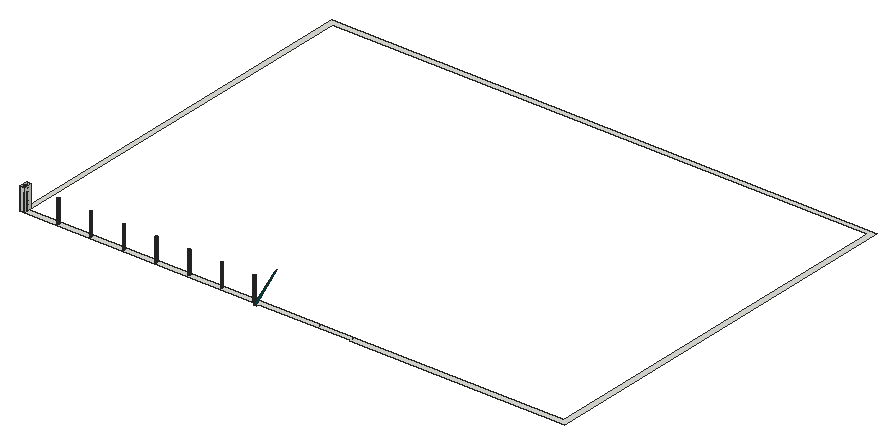
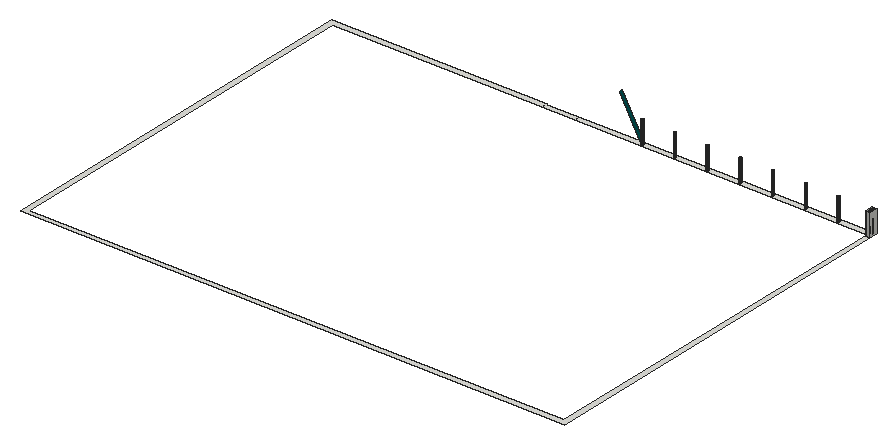
# SketchUp Ruby script. Lengths in inches.
U = 1.inch
M = Sketchup.active_model
def pt(a) = Geom::Point3d.new(a.map { |v| v * U })
def face(e, loops, mat)
  f = e.add_face(loops[0].map { |a| pt(a) })
  loops[1..].each { |l| e.add_face(l.map { |a| pt(a) }).erase! }
  f.material = f.back_material = mat if mat
  f
end
# faces: each face lists its corners as indices into pts; further lists are holes
def faces(e, pts, list, mat = nil) = list.each { |f| face(e, (f[0].is_a?(Array) ? f : [f]).map { |l| l.map { |i| pts[i] } }, mat) }
# xy, xz, yz: faces in a plane at the given z, y or x. An outline is a flat list of corners, or four numbers for a rectangle; further outlines are holes
def ring(l) = l.size == 4 ? [[l[0], l[1]], [l[2], l[1]], [l[2], l[3]], [l[0], l[3]]] : l.each_slice(2).to_a
def flat(e, list, mat, &to3) = list.each { |f| face(e, (f[0].is_a?(Array) ? f : [f]).map { |l| ring(l).map { |u, v| to3.(u, v) } }, mat) }
def xy(e, z, list, mat = nil) = flat(e, list, mat) { |x, y| [x, y, z] }
def xz(e, y, list, mat = nil) = flat(e, list, mat) { |x, z| [x, y, z] }
def yz(e, x, list, mat = nil) = flat(e, list, mat) { |y, z| [x, y, z] }
def lines(e, pts, list) = list.each { |a, b| e.add_line(pt(pts[a]), pt(pts[b])) }
# prism: a flat outline (further loops are holes) pulled along v
def prism(e, loops, v, mat = nil)
  f = face(e, loops, mat); d = Geom::Vector3d.new(v.map { |x| x * U })
  f.pushpull(f.normal.samedirection?(d) ? d.length : -d.length)
end
def box(e, o, s, mat = nil) = prism(e, [[o, [o[0] + s[0], o[1], o[2]], [o[0] + s[0], o[1] + s[1], o[2]], [o[0], o[1] + s[1], o[2]]]], [0, 0, s[2]], mat)
def at(x, y, z, deg = 0) = Geom::Transformation.translation(pt([x, y, z])) * Geom::Transformation.rotation(ORIGIN, Z_AXIS, deg.degrees)
def axes(o, x, y, z) = Geom::Transformation.new([*x, 0, *y, 0, *z, 0, *pt(o).to_a, 1])
def part(name) = M.definitions.add(name)
# library, detail: a bought-in or finely detailed component or shape, given as its bounding box
def library(name, o, s) = part(name).tap { |d| box(d.entities, o, s) }
def detail(e, o, s) = box(e.add_group.entities, o, s)
def put(e, d, t, mat = nil) = e.add_instance(d, t).tap { |i| i.material = mat if mat }
def group(e, t, mat = nil) = e.add_group.tap { |g| g.transformation = t; g.material = mat if mat }.entities
root = M.entities
M.materials.add("[0136_Charcoal]").color = [35, 35, 35]
M.materials.add("[Color H08]").color = [0, 102, 102]
xy(root,420,[[[426.66,30,430.89,30,430.89,36,595.0625,36,595.0625,35.0625,982.625,35.0625,982.625,738,0,738,0,49.95,8.62,49.95,8.62,36,426.66,36],[604.0625,44.0625,604.0625,45,9,45,9,729,973.625,729,973.625,44.0625],[973.58,39.3,973.09,39.36,972.64,39.55,972.25,39.85,971.96,40.24,971.77,40.6875,971.7,41.17,971.77,41.66,971.96,42.11,972.25,42.5,972.64,42.8,973.09,42.98,973.58,43.05,974.06,42.98,974.52,42.8,974.91,42.5,975.2,42.11,975.39,41.66,975.45,41.17,975.39,40.6875,975.2,40.24,974.91,39.85,974.52,39.55,974.06,39.36],[890.27,39.3,889.78,39.36,889.33,39.55,888.94,39.85,888.64,40.24,888.46,40.6875,888.39,41.17,888.46,41.66,888.64,42.11,888.94,42.5,889.33,42.8,889.78,42.98,890.27,43.05,890.75,42.98,891.2,42.8,891.59,42.5,891.89,42.11,892.08,41.66,892.14,41.17,892.08,40.6875,891.89,40.24,891.59,39.85,891.2,39.55,890.75,39.36],[831.27,39.3,830.78,39.36,830.33,39.55,829.94,39.85,829.64,40.24,829.46,40.6875,829.39,41.17,829.46,41.66,829.64,42.11,829.94,42.5,830.33,42.8,830.78,42.98,831.27,43.05,831.75,42.98,832.2,42.8,832.59,42.5,832.89,42.11,833.08,41.66,833.14,41.17,833.08,40.6875,832.89,40.24,832.59,39.85,832.2,39.55,831.75,39.36],[772.27,39.3,771.78,39.36,771.33,39.55,770.94,39.85,770.64,40.24,770.46,40.6875,770.39,41.17,770.46,41.66,770.64,42.11,770.94,42.5,771.33,42.8,771.78,42.98,772.27,43.05,772.75,42.98,773.2,42.8,773.59,42.5,773.89,42.11,774.08,41.66,774.14,41.17,774.08,40.6875,773.89,40.24,773.59,39.85,773.2,39.55,772.75,39.36],[713.27,39.3,712.78,39.36,712.33,39.55,711.94,39.85,711.64,40.24,711.46,40.6875,711.39,41.17,711.46,41.66,711.64,42.11,711.94,42.5,712.33,42.8,712.78,42.98,713.27,43.05,713.75,42.98,714.2,42.8,714.59,42.5,714.89,42.11,715.08,41.66,715.14,41.17,715.08,40.6875,714.89,40.24,714.59,39.85,714.2,39.55,713.75,39.36],[654.27,39.3,653.78,39.36,653.33,39.55,652.94,39.85,652.64,40.24,652.46,40.6875,652.39,41.17,652.46,41.66,652.64,42.11,652.94,42.5,653.33,42.8,653.78,42.98,654.27,43.05,654.75,42.98,655.2,42.8,655.59,42.5,655.89,42.11,656.08,41.66,656.14,41.17,656.08,40.6875,655.89,40.24,655.59,39.85,655.2,39.55,654.75,39.36],[595.27,39.3,594.78,39.36,594.33,39.55,593.94,39.85,593.64,40.24,593.46,40.6875,593.39,41.17,593.46,41.66,593.64,42.11,593.94,42.5,594.33,42.8,594.78,42.98,595.27,43.05,595.75,42.98,596.2,42.8,596.59,42.5,596.89,42.11,597.08,41.66,597.14,41.17,597.08,40.6875,596.89,40.24,596.59,39.85,596.2,39.55,595.75,39.36],[536.27,39.3,535.78,39.36,535.33,39.55,534.94,39.85,534.64,40.24,534.46,40.6875,534.39,41.17,534.46,41.66,534.64,42.11,534.94,42.5,535.33,42.8,535.78,42.98,536.27,43.05,536.75,42.98,537.2,42.8,537.59,42.5,537.89,42.11,538.08,41.66,538.14,41.17,538.08,40.6875,537.89,40.24,537.59,39.85,537.2,39.55,536.75,39.36],[477.27,39.3,476.78,39.36,476.33,39.55,475.94,39.85,475.64,40.24,475.46,40.6875,475.39,41.17,475.46,41.66,475.64,42.11,475.94,42.5,476.33,42.8,476.78,42.98,477.27,43.05,477.75,42.98,478.2,42.8,478.59,42.5,478.89,42.11,479.08,41.66,479.14,41.17,479.08,40.6875,478.89,40.24,478.59,39.85,478.2,39.55,477.75,39.36],[418.27,39.3,417.78,39.36,417.33,39.55,416.94,39.85,416.64,40.24,416.46,40.6875,416.39,41.17,416.46,41.66,416.64,42.11,416.94,42.5,417.33,42.8,417.78,42.98,418.27,43.05,418.75,42.98,419.2,42.8,419.59,42.5,419.89,42.11,420.08,41.66,420.14,41.17,420.08,40.6875,419.89,40.24,419.59,39.85,419.2,39.55,418.75,39.36],[359.27,39.3,358.78,39.36,358.33,39.55,357.94,39.85,357.64,40.24,357.46,40.6875,357.39,41.17,357.46,41.66,357.64,42.11,357.94,42.5,358.33,42.8,358.78,42.98,359.27,43.05,359.75,42.98,360.2,42.8,360.59,42.5,360.89,42.11,361.08,41.66,361.14,41.17,361.08,40.6875,360.89,40.24,360.59,39.85,360.2,39.55,359.75,39.36],[300.27,39.3,299.78,39.36,299.33,39.55,298.94,39.85,298.64,40.24,298.46,40.6875,298.39,41.17,298.46,41.66,298.64,42.11,298.94,42.5,299.33,42.8,299.78,42.98,300.27,43.05,300.75,42.98,301.2,42.8,301.59,42.5,301.89,42.11,302.08,41.66,302.14,41.17,302.08,40.6875,301.89,40.24,301.59,39.85,301.2,39.55,300.75,39.36],[241.27,39.3,240.78,39.36,240.33,39.55,239.94,39.85,239.64,40.24,239.46,40.6875,239.39,41.17,239.46,41.66,239.64,42.11,239.94,42.5,240.33,42.8,240.78,42.98,241.27,43.05,241.75,42.98,242.2,42.8,242.59,42.5,242.89,42.11,243.08,41.66,243.14,41.17,243.08,40.6875,242.89,40.24,242.59,39.85,242.2,39.55,241.75,39.36],[182.27,39.3,181.78,39.36,181.33,39.55,180.94,39.85,180.64,40.24,180.46,40.6875,180.39,41.17,180.46,41.66,180.64,42.11,180.94,42.5,181.33,42.8,181.78,42.98,182.27,43.05,182.75,42.98,183.2,42.8,183.59,42.5,183.89,42.11,184.08,41.66,184.14,41.17,184.08,40.6875,183.89,40.24,183.59,39.85,183.2,39.55,182.75,39.36],[123.27,39.3,122.78,39.36,122.33,39.55,121.94,39.85,121.64,40.24,121.46,40.6875,121.39,41.17,121.46,41.66,121.64,42.11,121.94,42.5,122.33,42.8,122.78,42.98,123.27,43.05,123.75,42.98,124.2,42.8,124.59,42.5,124.89,42.11,125.08,41.66,125.14,41.17,125.08,40.6875,124.89,40.24,124.59,39.85,124.2,39.55,123.75,39.36],[64.27,39.3,63.78,39.36,63.33,39.55,62.94,39.85,62.64,40.24,62.46,40.6875,62.39,41.17,62.46,41.66,62.64,42.11,62.94,42.5,63.33,42.8,63.78,42.98,64.27,43.05,64.75,42.98,65.2,42.8,65.59,42.5,65.89,42.11,66.08,41.66,66.14,41.17,66.08,40.6875,65.89,40.24,65.59,39.85,65.2,39.55,64.75,39.36]],[[0,36,8.62,49.95],[5.27,39.3,5.75,39.36,6.2,39.55,6.59,39.85,6.89,40.24,7.08,40.6875,7.14,41.17,7.08,41.66,6.89,42.11,6.59,42.5,6.2,42.8,5.75,42.98,5.27,43.05,4.78,42.98,4.33,42.8,3.94,42.5,3.64,42.11,3.46,41.66,3.39,41.17,3.46,40.6875,3.64,40.24,3.94,39.85,4.33,39.55,4.78,39.36]],[64.27,39.3,63.78,39.36,63.33,39.55,62.94,39.85,62.64,40.24,62.46,40.6875,62.39,41.17,62.46,41.66,62.64,42.11,62.94,42.5,63.33,42.8,63.78,42.98,64.27,43.05,64.75,42.98,65.2,42.8,65.59,42.5,65.89,42.11,66.08,41.66,66.14,41.17,66.08,40.6875,65.89,40.24,65.59,39.85,65.2,39.55,64.75,39.36],[123.27,39.3,122.78,39.36,122.33,39.55,121.94,39.85,121.64,40.24,121.46,40.6875,121.39,41.17,121.46,41.66,121.64,42.11,121.94,42.5,122.33,42.8,122.78,42.98,123.27,43.05,123.75,42.98,124.2,42.8,124.59,42.5,124.89,42.11,125.08,41.66,125.14,41.17,125.08,40.6875,124.89,40.24,124.59,39.85,124.2,39.55,123.75,39.36],[182.27,39.3,181.78,39.36,181.33,39.55,180.94,39.85,180.64,40.24,180.46,40.6875,180.39,41.17,180.46,41.66,180.64,42.11,180.94,42.5,181.33,42.8,181.78,42.98,182.27,43.05,182.75,42.98,183.2,42.8,183.59,42.5,183.89,42.11,184.08,41.66,184.14,41.17,184.08,40.6875,183.89,40.24,183.59,39.85,183.2,39.55,182.75,39.36],
  [241.27,39.3,240.78,39.36,240.33,39.55,239.94,39.85,239.64,40.24,239.46,40.6875,239.39,41.17,239.46,41.66,239.64,42.11,239.94,42.5,240.33,42.8,240.78,42.98,241.27,43.05,241.75,42.98,242.2,42.8,242.59,42.5,242.89,42.11,243.08,41.66,243.14,41.17,243.08,40.6875,242.89,40.24,242.59,39.85,242.2,39.55,241.75,39.36],[300.27,39.3,299.78,39.36,299.33,39.55,298.94,39.85,298.64,40.24,298.46,40.6875,298.39,41.17,298.46,41.66,298.64,42.11,298.94,42.5,299.33,42.8,299.78,42.98,300.27,43.05,300.75,42.98,301.2,42.8,301.59,42.5,301.89,42.11,302.08,41.66,302.14,41.17,302.08,40.6875,301.89,40.24,301.59,39.85,301.2,39.55,300.75,39.36],[359.27,39.3,358.78,39.36,358.33,39.55,357.94,39.85,357.64,40.24,357.46,40.6875,357.39,41.17,357.46,41.66,357.64,42.11,357.94,42.5,358.33,42.8,358.78,42.98,359.27,43.05,359.75,42.98,360.2,42.8,360.59,42.5,360.89,42.11,361.08,41.66,361.14,41.17,361.08,40.6875,360.89,40.24,360.59,39.85,360.2,39.55,359.75,39.36],[418.27,39.3,417.78,39.36,417.33,39.55,416.94,39.85,416.64,40.24,416.46,40.6875,416.39,41.17,416.46,41.66,416.64,42.11,416.94,42.5,417.33,42.8,417.78,42.98,418.27,43.05,418.75,42.98,419.2,42.8,419.59,42.5,419.89,42.11,420.08,41.66,420.14,41.17,420.08,40.6875,419.89,40.24,419.59,39.85,419.2,39.55,418.75,39.36]])
xz(root,36,[[0,420,8.62,460.3125]])
xz(root,49.95,[[0,420,8.62,460.3125]])
yz(root,0,[[36,420,49.95,460.3125]])
yz(root,8.62,[[[36,420,49.95,460.3125],[41.84,455.4,41.36,455.46,40.91,455.65,40.52,455.95,40.22,456.34,40.03,456.79,39.97,457.28,40.03,457.76,40.22,458.21,40.52,458.6,40.91,458.9,41.36,459.09,41.84,459.15,42.33,459.09,42.78,458.9,43.17,458.6,43.47,458.21,43.66,457.76,43.72,457.28,43.66,456.79,43.47,456.34,43.17,455.95,42.78,455.65,42.33,455.46],[41.84,448.46,41.36,448.53,40.91,448.71,40.52,449.01,40.22,449.4,40.03,449.85,39.97,450.34,40.03,450.82,40.22,451.28,40.52,451.66,40.91,451.96,41.36,452.15,41.84,452.21,42.33,452.15,42.78,451.96,43.17,451.66,43.47,451.28,43.66,450.82,43.72,450.34,43.66,449.85,43.47,449.4,43.17,449.01,42.78,448.71,42.33,448.53],[41.84,441.53,41.36,441.59,40.91,441.78,40.52,442.07,40.22,442.46,40.03,442.92,39.97,443.4,40.03,443.89,40.22,444.34,40.52,444.73,40.91,445.02,41.36,445.21,41.84,445.28,42.33,445.21,42.78,445.02,43.17,444.73,43.47,444.34,43.66,443.89,43.72,443.4,43.66,442.92,43.47,442.46,43.17,442.07,42.78,441.78,42.33,441.59],[41.84,434.59,41.36,434.65,40.91,434.84,40.52,435.14,40.22,435.53,40.03,435.98,39.97,436.46,40.03,436.95,40.22,437.4,40.52,437.79,40.91,438.09,41.36,438.27,41.84,438.34,42.33,438.27,42.78,438.09,43.17,437.79,43.47,437.4,43.66,436.95,43.72,436.46,43.66,435.98,43.47,435.53,43.17,435.14,42.78,434.84,42.33,434.65],[41.84,427.65,41.36,427.71,40.91,427.9,40.52,428.2,40.22,428.59,40.03,429.04,39.97,429.53,40.03,430.01,40.22,430.46,40.52,430.85,40.91,431.15,41.36,431.34,41.84,431.4,42.33,431.34,42.78,431.15,43.17,430.85,43.47,430.46,43.66,430.01,43.72,429.53,43.66,429.04,43.47,428.59,43.17,428.2,42.78,427.9,42.33,427.71],[41.84,420.71,41.36,420.78,40.91,420.96,40.52,421.26,40.22,421.65,40.03,422.1,39.97,422.59,40.03,423.07,40.22,423.53,40.52,423.91,40.91,424.21,41.36,424.4,41.84,424.46,42.33,424.4,42.78,424.21,43.17,423.91,43.47,423.53,43.66,423.07,43.72,422.59,43.66,422.1,43.47,421.65,43.17,421.26,42.78,420.96,42.33,420.78]]])
p = [[463.18,36,486.6875],[426.66,36,420],[426.66,30,420],[463.18,30,486.6875],[4.78,39.36,420],[5.27,39.3,420],
  [5.27,39.3,460.3125],[4.78,39.36,460.3125],[5.75,39.36,420],[5.75,39.36,460.3125],[63.78,39.36,420],[64.27,39.3,420],
  [64.27,39.3,460.3125],[63.78,39.36,460.3125],[64.75,39.36,420],[64.75,39.36,460.3125],[122.78,39.36,420],[123.27,39.3,420],
  [123.27,39.3,460.3125],[122.78,39.36,460.3125],[123.75,39.36,420],[123.75,39.36,460.3125],[181.78,39.36,420],[182.27,39.3,420],
  [182.27,39.3,460.3125],[181.78,39.36,460.3125],[182.75,39.36,420],[182.75,39.36,460.3125],[240.78,39.36,420],[241.27,39.3,420],
  [241.27,39.3,460.3125],[240.78,39.36,460.3125],[241.75,39.36,420],[241.75,39.36,460.3125],[299.78,39.36,420],[300.27,39.3,420],
  [300.27,39.3,460.3125],[299.78,39.36,460.3125],[300.75,39.36,420],[300.75,39.36,460.3125],[358.78,39.36,420],[359.27,39.3,420],
  [359.27,39.3,460.3125],[358.78,39.36,460.3125],[359.75,39.36,420],[359.75,39.36,460.3125],[417.78,39.36,420],[418.27,39.3,420],
  [418.27,39.3,460.3125],[417.78,39.36,460.3125],[418.75,39.36,420],[418.75,39.36,460.3125],[4.33,39.55,420],[4.33,39.55,460.3125],
  [6.2,39.55,420],[6.2,39.55,460.3125],[63.33,39.55,420],[63.33,39.55,460.3125],[65.2,39.55,420],[65.2,39.55,460.3125],
  [122.33,39.55,420],[122.33,39.55,460.3125],[124.2,39.55,420],[124.2,39.55,460.3125],[181.33,39.55,420],[181.33,39.55,460.3125],
  [183.2,39.55,420],[183.2,39.55,460.3125],[240.33,39.55,420],[240.33,39.55,460.3125],[242.2,39.55,420],[242.2,39.55,460.3125],
  [299.33,39.55,420],[299.33,39.55,460.3125],[301.2,39.55,420],[301.2,39.55,460.3125],[358.33,39.55,420],[358.33,39.55,460.3125],
  [360.2,39.55,420],[360.2,39.55,460.3125],[417.33,39.55,420],[417.33,39.55,460.3125],[419.2,39.55,420],[419.2,39.55,460.3125],
  [3.94,39.85,420],[3.94,39.85,460.3125],[6.59,39.85,420],[6.59,39.85,460.3125],[62.94,39.85,420],[62.94,39.85,460.3125],
  [65.59,39.85,420],[65.59,39.85,460.3125],[121.94,39.85,420],[121.94,39.85,460.3125],[124.59,39.85,420],[124.59,39.85,460.3125],
  [180.94,39.85,420],[180.94,39.85,460.3125],[183.59,39.85,420],[183.59,39.85,460.3125],[239.94,39.85,420],[239.94,39.85,460.3125],
  [242.59,39.85,420],[242.59,39.85,460.3125],[298.94,39.85,420],[298.94,39.85,460.3125],[301.59,39.85,420],[301.59,39.85,460.3125],
  [357.94,39.85,420],[357.94,39.85,460.3125],[360.59,39.85,420],[360.59,39.85,460.3125],[416.94,39.85,420],[416.94,39.85,460.3125],
  [419.59,39.85,420],[419.59,39.85,460.3125],[3.64,40.24,420],[3.64,40.24,460.3125],[6.89,40.24,420],[6.89,40.24,460.3125],
  [62.64,40.24,420],[62.64,40.24,460.3125],[65.89,40.24,420],[65.89,40.24,460.3125],[121.64,40.24,420],[121.64,40.24,460.3125],
  [124.89,40.24,420],[124.89,40.24,460.3125],[180.64,40.24,420],[180.64,40.24,460.3125],[183.89,40.24,420],[183.89,40.24,460.3125],
  [239.64,40.24,420],[239.64,40.24,460.3125],[242.89,40.24,420],[242.89,40.24,460.3125],[298.64,40.24,420],[298.64,40.24,460.3125],
  [301.89,40.24,420],[301.89,40.24,460.3125],[357.64,40.24,420],[357.64,40.24,460.3125],[360.89,40.24,420],[360.89,40.24,460.3125],
  [416.64,40.24,420],[416.64,40.24,460.3125],[419.89,40.24,420],[419.89,40.24,460.3125],[3.46,40.6875,420],[3.46,40.6875,460.3125],
  [7.08,40.6875,420],[7.08,40.6875,460.3125],[62.46,40.6875,420],[62.46,40.6875,460.3125],[66.08,40.6875,420],[66.08,40.6875,460.3125],
  [121.46,40.6875,420],[121.46,40.6875,460.3125],[125.08,40.6875,420],[125.08,40.6875,460.3125],[180.46,40.6875,420],[180.46,40.6875,460.3125],
  [184.08,40.6875,420],[184.08,40.6875,460.3125],[239.46,40.6875,420],[239.46,40.6875,460.3125],[243.08,40.6875,420],[243.08,40.6875,460.3125],
  [298.46,40.6875,420],[298.46,40.6875,460.3125],[302.08,40.6875,420],[302.08,40.6875,460.3125],[357.46,40.6875,420],[357.46,40.6875,460.3125],
  [361.08,40.6875,420],[361.08,40.6875,460.3125],[416.46,40.6875,420],[416.46,40.6875,460.3125],[420.08,40.6875,420],[420.08,40.6875,460.3125],
  [3.39,41.17,420],[3.39,41.17,460.3125],[7.14,41.17,420],[7.14,41.17,460.3125],[62.39,41.17,420],[62.39,41.17,460.3125],
  [66.14,41.17,420],[66.14,41.17,460.3125],[121.39,41.17,420],[121.39,41.17,460.3125],[125.14,41.17,420],[125.14,41.17,460.3125],
  [180.39,41.17,420],[180.39,41.17,460.3125],[184.14,41.17,420],[184.14,41.17,460.3125],[239.39,41.17,420],[239.39,41.17,460.3125],
  [243.14,41.17,420],[243.14,41.17,460.3125],[298.39,41.17,420],[298.39,41.17,460.3125],[302.14,41.17,420],[302.14,41.17,460.3125],
  [357.39,41.17,420],[357.39,41.17,460.3125],[361.14,41.17,420],[361.14,41.17,460.3125],[416.39,41.17,420],[416.39,41.17,460.3125],
  [420.14,41.17,420],[420.14,41.17,460.3125],[3.46,41.66,420],[3.46,41.66,460.3125],[7.08,41.66,420],[7.08,41.66,460.3125],
  [62.46,41.66,420],[62.46,41.66,460.3125],[66.08,41.66,420],[66.08,41.66,460.3125],[121.46,41.66,420],[121.46,41.66,460.3125],
  [125.08,41.66,420],[125.08,41.66,460.3125],[180.46,41.66,420],[180.46,41.66,460.3125],[184.08,41.66,420],[184.08,41.66,460.3125],
  [239.46,41.66,420],[239.46,41.66,460.3125],[243.08,41.66,420],[243.08,41.66,460.3125],[298.46,41.66,420],[298.46,41.66,460.3125],
  [302.08,41.66,420],[302.08,41.66,460.3125],[357.46,41.66,420],[357.46,41.66,460.3125],[361.08,41.66,420],[361.08,41.66,460.3125],
  [416.46,41.66,420],[416.46,41.66,460.3125],[420.08,41.66,420],[420.08,41.66,460.3125],[3.64,42.11,420],[3.64,42.11,460.3125],
  [6.89,42.11,420],[6.89,42.11,460.3125],[62.64,42.11,420],[62.64,42.11,460.3125],[65.89,42.11,420],[65.89,42.11,460.3125],
  [121.64,42.11,420],[121.64,42.11,460.3125],[124.89,42.11,420],[124.89,42.11,460.3125],[180.64,42.11,420],[180.64,42.11,460.3125],
  [183.89,42.11,420],[183.89,42.11,460.3125],[239.64,42.11,420],[239.64,42.11,460.3125],[242.89,42.11,420],[242.89,42.11,460.3125],
  [298.64,42.11,420],[298.64,42.11,460.3125],[301.89,42.11,420],[301.89,42.11,460.3125],[357.64,42.11,420],[357.64,42.11,460.3125],
  [360.89,42.11,420],[360.89,42.11,460.3125],[416.64,42.11,420],[416.64,42.11,460.3125],[419.89,42.11,420],[419.89,42.11,460.3125],
  [3.94,42.5,420],[3.94,42.5,460.3125],[6.59,42.5,420],[6.59,42.5,460.3125],[62.94,42.5,420],[62.94,42.5,460.3125],
  [65.59,42.5,420],[65.59,42.5,460.3125],[121.94,42.5,420],[121.94,42.5,460.3125],[124.59,42.5,420],[124.59,42.5,460.3125],
  [180.94,42.5,420],[180.94,42.5,460.3125],[183.59,42.5,420],[183.59,42.5,460.3125],[239.94,42.5,420],[239.94,42.5,460.3125],
  [242.59,42.5,420],[242.59,42.5,460.3125],[298.94,42.5,420],[298.94,42.5,460.3125],[301.59,42.5,420],[301.59,42.5,460.3125],
  [357.94,42.5,420],[357.94,42.5,460.3125],[360.59,42.5,420],[360.59,42.5,460.3125],[416.94,42.5,420],[416.94,42.5,460.3125],
  [419.59,42.5,420],[419.59,42.5,460.3125],[4.33,42.8,420],[4.33,42.8,460.3125],[6.2,42.8,420],[6.2,42.8,460.3125],
  [63.33,42.8,420],[63.33,42.8,460.3125],[65.2,42.8,420],[65.2,42.8,460.3125],[122.33,42.8,420],[122.33,42.8,460.3125],
  [124.2,42.8,420],[124.2,42.8,460.3125],[181.33,42.8,420],[181.33,42.8,460.3125],[183.2,42.8,420],[183.2,42.8,460.3125],
  [240.33,42.8,420],[240.33,42.8,460.3125],[242.2,42.8,420],[242.2,42.8,460.3125],[299.33,42.8,420],[299.33,42.8,460.3125],
  [301.2,42.8,420],[301.2,42.8,460.3125],[358.33,42.8,420],[358.33,42.8,460.3125],[360.2,42.8,420],[360.2,42.8,460.3125],
  [417.33,42.8,420],[417.33,42.8,460.3125],[419.2,42.8,420],[419.2,42.8,460.3125],[4.78,42.98,420],[4.78,42.98,460.3125],
  [5.75,42.98,420],[5.75,42.98,460.3125],[63.78,42.98,420],[63.78,42.98,460.3125],[64.75,42.98,420],[64.75,42.98,460.3125],
  [122.78,42.98,420],[122.78,42.98,460.3125],[123.75,42.98,420],[123.75,42.98,460.3125],[181.78,42.98,420],[181.78,42.98,460.3125],
  [182.75,42.98,420],[182.75,42.98,460.3125],[240.78,42.98,420],[240.78,42.98,460.3125],[241.75,42.98,420],[241.75,42.98,460.3125],
  [299.78,42.98,420],[299.78,42.98,460.3125],[300.75,42.98,420],[300.75,42.98,460.3125],[358.78,42.98,420],[358.78,42.98,460.3125],
  [359.75,42.98,420],[359.75,42.98,460.3125],[417.78,42.98,420],[417.78,42.98,460.3125],[418.75,42.98,420],[418.75,42.98,460.3125],
  [5.27,43.05,420],[5.27,43.05,460.3125],[64.27,43.05,420],[64.27,43.05,460.3125],[123.27,43.05,420],[123.27,43.05,460.3125],
  [182.27,43.05,420],[182.27,43.05,460.3125],[241.27,43.05,420],[241.27,43.05,460.3125],[300.27,43.05,420],[300.27,43.05,460.3125],
  [359.27,43.05,420],[359.27,43.05,460.3125],[418.27,43.05,420],[418.27,43.05,460.3125]]
faces(root,p,[[0,1,2,3]],"[Color H08]")
faces(root,p,[[4,5,6,7],[5,8,9,6],[52,4,7,53],[8,54,55,9],[84,52,53,85],[54,86,87,55],[116,84,85,117],[86,118,119,87],
  [148,116,117,149],[118,150,151,119],[180,148,149,181],[150,182,183,151],[212,180,181,213],[182,214,215,183],[244,212,213,245],[214,246,247,215],
  [276,244,245,277],[246,278,279,247],[308,276,277,309],[278,310,311,279],[340,308,309,341],[310,342,343,311],[372,340,341,373],[342,372,373,343]])
faces(root,p,[[10,11,12,13],[11,14,15,12],[16,17,18,19],[17,20,21,18],[22,23,24,25],[23,26,27,24],[28,29,30,31],[29,32,33,30],
  [34,35,36,37],[35,38,39,36],[40,41,42,43],[41,44,45,42],[46,47,48,49],[47,50,51,48],[56,10,13,57],[14,58,59,15],
  [60,16,19,61],[20,62,63,21],[64,22,25,65],[26,66,67,27],[68,28,31,69],[32,70,71,33],[72,34,37,73],[38,74,75,39],
  [76,40,43,77],[44,78,79,45],[80,46,49,81],[50,82,83,51],[88,56,57,89],[58,90,91,59],[92,60,61,93],[62,94,95,63],
  [96,64,65,97],[66,98,99,67],[100,68,69,101],[70,102,103,71],[104,72,73,105],[74,106,107,75],[108,76,77,109],[78,110,111,79],
  [112,80,81,113],[82,114,115,83],[120,88,89,121],[90,122,123,91],[124,92,93,125],[94,126,127,95],[128,96,97,129],[98,130,131,99],
  [132,100,101,133],[102,134,135,103],[136,104,105,137],[106,138,139,107],[140,108,109,141],[110,142,143,111],[144,112,113,145],[114,146,147,115],
  [152,120,121,153],[122,154,155,123],[156,124,125,157],[126,158,159,127],[160,128,129,161],[130,162,163,131],[164,132,133,165],[134,166,167,135],
  [168,136,137,169],[138,170,171,139],[172,140,141,173],[142,174,175,143],[176,144,145,177],[146,178,179,147],[184,152,153,185],[154,186,187,155],
  [188,156,157,189],[158,190,191,159],[192,160,161,193],[162,194,195,163],[196,164,165,197],[166,198,199,167],[200,168,169,201],[170,202,203,171],
  [204,172,173,205],[174,206,207,175],[208,176,177,209],[178,210,211,179],[216,184,185,217],[186,218,219,187],[220,188,189,221],[190,222,223,191],
  [224,192,193,225],[194,226,227,195],[228,196,197,229],[198,230,231,199],[232,200,201,233],[202,234,235,203],[236,204,205,237],[206,238,239,207],
  [240,208,209,241],[210,242,243,211],[248,216,217,249],[218,250,251,219],[252,220,221,253],[222,254,255,223],[256,224,225,257],[226,258,259,227],
  [260,228,229,261],[230,262,263,231],[264,232,233,265],[234,266,267,235],[268,236,237,269],[238,270,271,239],[272,240,241,273],[242,274,275,243],
  [280,248,249,281],[250,282,283,251],[284,252,253,285],[254,286,287,255],[288,256,257,289],[258,290,291,259],[292,260,261,293],[262,294,295,263],
  [296,264,265,297],[266,298,299,267],[300,268,269,301],[270,302,303,271],[304,272,273,305],[274,306,307,275],[312,280,281,313],[282,314,315,283],
  [316,284,285,317],[286,318,319,287],[320,288,289,321],[290,322,323,291],[324,292,293,325],[294,326,327,295],[328,296,297,329],[298,330,331,299],
  [332,300,301,333],[302,334,335,303],[336,304,305,337],[306,338,339,307],[344,312,313,345],[314,346,347,315],[348,316,317,349],[318,350,351,319],
  [352,320,321,353],[322,354,355,323],[356,324,325,357],[326,358,359,327],[360,328,329,361],[330,362,363,331],[364,332,333,365],[334,366,367,335],
  [368,336,337,369],[338,370,371,339],[374,344,345,375],[346,374,375,347],[376,348,349,377],[350,376,377,351],[378,352,353,379],[354,378,379,355],
  [380,356,357,381],[358,380,381,359],[382,360,361,383],[362,382,383,363],[384,364,365,385],[366,384,385,367],[386,368,369,387],[370,386,387,371]],"[0136_Charcoal]")
